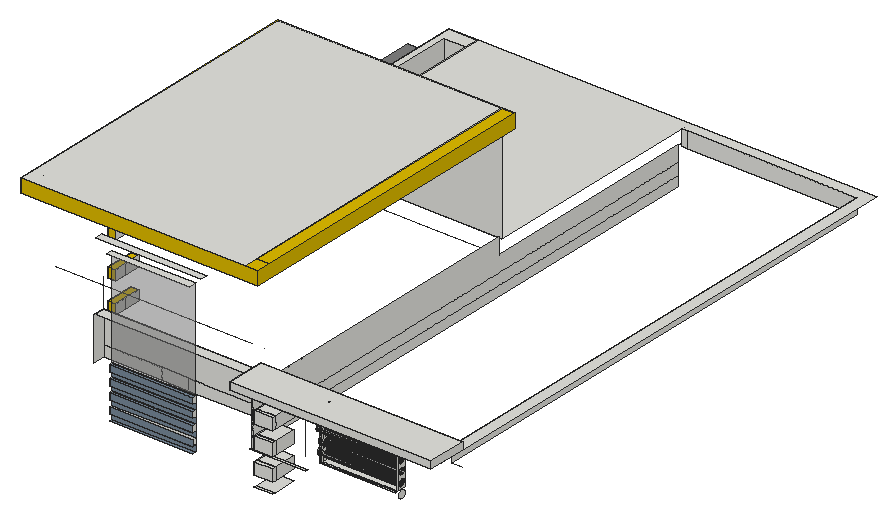
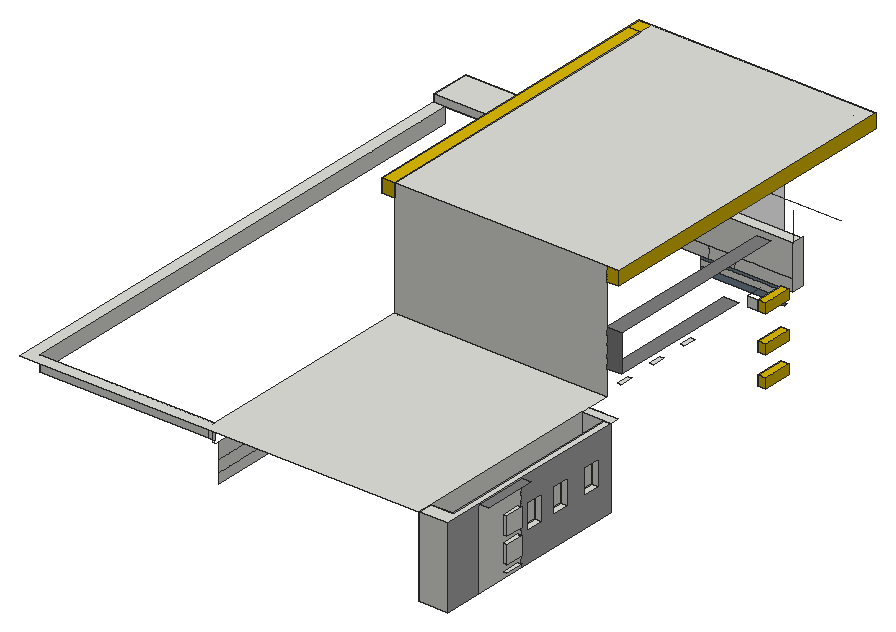
# SketchUp Ruby script. Lengths in inches.
U = 1.inch
M = Sketchup.active_model
def pt(a) = Geom::Point3d.new(a.map { |v| v * U })
def face(e, loops, mat)
  f = e.add_face(loops[0].map { |a| pt(a) })
  loops[1..].each { |l| e.add_face(l.map { |a| pt(a) }).erase! }
  f.material = f.back_material = mat if mat
  f
end
# faces: each face lists its corners as indices into pts; further lists are holes
def faces(e, pts, list, mat = nil) = list.each { |f| face(e, (f[0].is_a?(Array) ? f : [f]).map { |l| l.map { |i| pts[i] } }, mat) }
# xy, xz, yz: faces in a plane at the given z, y or x. An outline is a flat list of corners, or four numbers for a rectangle; further outlines are holes
def ring(l) = l.size == 4 ? [[l[0], l[1]], [l[2], l[1]], [l[2], l[3]], [l[0], l[3]]] : l.each_slice(2).to_a
def flat(e, list, mat, &to3) = list.each { |f| face(e, (f[0].is_a?(Array) ? f : [f]).map { |l| ring(l).map { |u, v| to3.(u, v) } }, mat) }
def xy(e, z, list, mat = nil) = flat(e, list, mat) { |x, y| [x, y, z] }
def xz(e, y, list, mat = nil) = flat(e, list, mat) { |x, z| [x, y, z] }
def yz(e, x, list, mat = nil) = flat(e, list, mat) { |y, z| [x, y, z] }
def lines(e, pts, list) = list.each { |a, b| e.add_line(pt(pts[a]), pt(pts[b])) }
# prism: a flat outline (further loops are holes) pulled along v
def prism(e, loops, v, mat = nil)
  f = face(e, loops, mat); d = Geom::Vector3d.new(v.map { |x| x * U })
  f.pushpull(f.normal.samedirection?(d) ? d.length : -d.length)
end
def box(e, o, s, mat = nil) = prism(e, [[o, [o[0] + s[0], o[1], o[2]], [o[0] + s[0], o[1] + s[1], o[2]], [o[0], o[1] + s[1], o[2]]]], [0, 0, s[2]], mat)
def at(x, y, z, deg = 0) = Geom::Transformation.translation(pt([x, y, z])) * Geom::Transformation.rotation(ORIGIN, Z_AXIS, deg.degrees)
def axes(o, x, y, z) = Geom::Transformation.new([*x, 0, *y, 0, *z, 0, *pt(o).to_a, 1])
def part(name) = M.definitions.add(name)
# library, detail: a bought-in or finely detailed component or shape, given as its bounding box
def library(name, o, s) = part(name).tap { |d| box(d.entities, o, s) }
def detail(e, o, s) = box(e.add_group.entities, o, s)
def put(e, d, t, mat = nil) = e.add_instance(d, t).tap { |i| i.material = mat if mat }
def group(e, t, mat = nil) = e.add_group.tap { |g| g.transformation = t; g.material = mat if mat }.entities
root = M.entities
M.materials.add("[0046_Gold]").color = [221, 186, 0]
M.materials.add("[0110_LightSlateGray]").color = [119, 136, 153]
M.materials.add("[0132_LightGray]").color = [169, 169, 169]
M.materials.add("[0133_Gray]").color = [128, 128, 128]
M.materials.add("[Translucent Glass Gray]").color = [128, 128, 128]
M.materials["[Translucent Glass Gray]"].alpha = 0.5
xy(root,272.6,[[82,329.95,87.58,329.95,87.58,486.08,106,486.08,106,494.21,82,494.21],[87.58,329.95,106,486.08],[82,494.21,106,498.31]])
xy(root,273.2,[[288.75,38.62,303.875,41.62],[288.75,41.62,303.875,61.06]])
xy(root,274.59,[[162.79,46.06,231.72,49.06]],"[0110_LightSlateGray]")
xy(root,280.11,[[162.79,46.06,231.72,49.06]],"[0110_LightSlateGray]")
xy(root,282.14,[[288.75,38.62,303.875,41.62],[288.75,41.62,303.875,61.06]])
xy(root,285.27,[[70.87,436.12,73.87,451.12]])
xy(root,289.0625,[[88,138.31,94,162.08]],"[0046_Gold]")
xy(root,290.55,[[162.79,46.06,231.72,49.06]],"[0110_LightSlateGray]")
xy(root,291.33,[[70.87,436.12,73.87,451.12]])
xy(root,292.2,[[288.75,38.62,303.875,41.62],[288.75,41.62,303.875,61.06]])
xy(root,294.8125,[[279.43,45.87,325.52,47.62],[325.52,60.18,326.02,61.06],[326.02,60.18,388.7,61.06],[325.52,61.06,326.02,70.06],[326.02,61.06,388.7,62.68],
  [326.02,62.68,388.7,70.06]])
xy(root,295.46,[[162.79,46.06,231.72,49.06]],"[0110_LightSlateGray]")
xy(root,297.34,[[88,138.31,94,162.08]],"[0046_Gold]")
xy(root,297.7,[[82,342.29,87.58,357.98],[82,374.54,87.58,390.23],[82,401.35,87.58,417.04]])
xy(root,300.98,[[162.79,46.06,231.72,49.06]],"[0110_LightSlateGray]")
xy(root,301.14,[[288.75,38.62,303.875,41.62],[288.75,41.62,303.875,61.06]])
xy(root,305.9,[[162.79,46.06,231.72,49.06]],"[0110_LightSlateGray]")
xy(root,306.33,[[70.87,436.12,73.87,451.12]])
xy(root,311.2,[[288.75,38.62,303.875,41.62],[288.75,41.62,303.875,61.06]])
xy(root,311.42,[[162.79,46.06,231.72,49.06]],"[0110_LightSlateGray]")
xy(root,312.39,[[70.87,436.12,73.87,451.12]])
xy(root,314.34,[[88,138.31,94,162.08]],"[0046_Gold]")
xy(root,316.34,[[162.79,46.06,231.72,49.06]],"[0110_LightSlateGray]")
xy(root,318.45,[[82,342.29,87.58,357.98],[82,374.54,87.58,390.23],[82,401.35,87.58,417.04]])
xy(root,320.14,[[288.75,38.62,303.875,41.62],[288.75,41.62,303.875,61.06]])
xy(root,322.62,[[88,138.31,94,162.08]],"[0046_Gold]")
xy(root,327.39,[[70.87,436.12,73.87,451.12]])
xy(root,330.2,[[288.75,38.62,303.875,41.62],[288.75,41.62,303.875,61.06]])
xy(root,339,[[269.16,37.37,326.02,41.62],[326.02,37.37,326.02,70.06,388.7,70.06,388.7,47.37,411.96,47.37,411.96,55.06,416.22,55.06,416.22,47.37,436.31,47.37,436.31,37.37],[269.16,41.62,279.47,47.62],[279.47,41.62,288.87,47.62],[288.87,41.62,326.02,47.62],
  [388.7,47.37,411.96,61.68],[416.22,47.37,427.31,48.18],[427.31,47.37,436.31,48.18],[269.16,47.62,279.43,49.06],[279.43,47.62,279.47,49.06],
  [279.47,47.62,288.87,47.62,288.87,56.62,287.5,56.62,287.5,49.06,282.09,49.06,282.09,56.62,279.47,56.62],[288.87,47.62,325.52,56.62],[325.52,47.62,326.02,56.62],[416.22,48.18,427.31,61.06],[427.31,48.18,436.31,61.06],
  [269.16,49.06,279.43,56.62],[279.43,49.06,279.47,56.62],[282.09,49.06,287.5,56.62],[282.09,49.06,287.5,56.62],[411.96,55.06,416.22,61.06],
  [269.16,56.62,279.43,61.06],[279.43,56.62,279.47,60.18],[279.47,56.62,282.09,60.18],[282.09,56.62,287.5,60.18],[287.5,56.62,288.87,60.18],
  [288.87,56.62,325.52,60.18],[325.52,56.62,326.02,60.18],[279.43,60.18,279.47,61.06],[279.47,60.18,282.09,60.81],[282.09,60.18,287.5,60.81],
  [287.5,60.18,288.87,60.81],[288.87,60.18,325.52,60.81],[325.52,60.18,326.02,60.81],[279.47,60.81,282.09,61.06],[282.09,60.81,287.5,61.06],
  [287.5,60.81,288.87,61.06],[288.87,60.81,313.39,61.06],[313.39,60.81,325.52,61.06],[325.52,60.81,326.02,61.06],[138.64,61.06,269.16,70.06],
  [269.16,61.06,279.43,70.06],[279.43,61.06,279.47,70.06],[279.47,61.06,282.09,61.18],[282.09,61.06,287.5,61.18],[287.5,61.06,288.87,61.18],
  [288.87,61.06,313.39,61.18],[313.39,61.06,325.52,61.18],[325.52,61.06,326.02,61.18],[411.96,61.06,416.22,62.68],[416.22,61.06,427.31,62.68],
  [427.31,61.06,436.31,70.06],[279.47,61.18,282.09,61.31],[282.09,61.18,287.5,61.31],[287.5,61.18,288.87,61.31],[288.87,61.18,313.39,61.31],
  [313.39,61.18,325.52,61.31],[325.52,61.18,326.02,61.31],[279.47,61.31,282.09,62.68],[282.09,61.31,287.5,62.68],[287.5,61.31,288.87,62.68],
  [288.87,61.31,313.39,62.68],[313.39,61.31,325.52,62.68],[325.52,61.31,326.02,62.68],[388.7,61.68,411.96,62.68],[279.47,62.68,282.09,70.06],
  [282.09,62.68,287.5,70.06],[287.5,62.68,313.39,70.06],[313.39,62.68,325.52,70.06],[325.52,62.68,326.02,70.06],[388.7,62.68,411.96,70.06],
  [411.96,62.68,416.22,70.06],[416.22,62.68,427.31,70.06],[427.31,70.06,436.31,70.06,436.31,498.31,106,498.31,106,303.56,282.09,303.56,282.09,489.31,427.31,489.31],[279.43,70.06,279.47,303.56],[82,322.08,106,329.95],
  [82,329.95,87.58,329.95,87.58,486.08,106,486.08,106,498.31,82,498.31]])
xy(root,339,[[73.87,422.6,82,466.21]],"[0133_Gray]")
xy(root,341.65,[[106,212.89,109,223.64],[106,244.77,109,255.52],[106,278.27,109,289.02]])
xy(root,344.71,[[88,138.31,94,162.08]],"[0046_Gold]")
xy(root,345,[[269.16,37.37,436.31,70.06]])
xy(root,352.99,[[88,138.31,94,162.08]],"[0046_Gold]")
xy(root,359.72,[[94,182.43,106,303.56]],"[0133_Gray]")
xy(root,390.53,[[94,148.68,106,303.56]],"[0133_Gray]")
xy(root,399.9,[[162.79,43.06,231.72,49.06]])
xy(root,408.9,[[153.79,43.06,240.72,49.06]])
xy(root,424.32,[[103,82.06,106,90.88],[103,99.88,106,108.69],[103,116.44,106,125.25],[106,116.44,109,125.25]])
xy(root,424.32,[[96.18,37.06,96.18,303.56,106,303.56,106,125.25,103,125.25,103,116.44,106,116.44,106,108.69,103,108.69,103,99.88,106,99.88,106,90.88,103,90.88,103,82.06,106,82.06,106,49.06,282.09,49.06,282.09,303.56,292.72,303.56,292.72,37.06]],"[0046_Gold]")
xy(root,435.8125,[[96.18,37.06,282.09,303.56]])
xy(root,435.8125,[[282.09,37.06,292.72,49.06],[282.09,49.06,292.72,303.56]],"[0046_Gold]")
xz(root,37.06,[[96.18,424.32,292.72,435.8125]],"[0046_Gold]")
xz(root,37.37,[[269.16,339,436.31,345]])
xz(root,38.62,[[288.75,282.14,303.875,292.2],[288.75,301.14,303.875,311.2],[288.75,320.14,303.875,330.2]])
xz(root,41.62,[[288.75,282.14,303.875,292.2],[288.75,301.14,303.875,311.2],[288.75,320.14,303.875,330.2]])
xz(root,46.06,[[162.79,280.11,231.72,285.03],[162.79,290.55,231.72,295.46],[162.79,300.98,231.72,305.9],[162.79,311.42,231.72,316.34]],"[0110_LightSlateGray]")
xz(root,49.06,[[162.79,280.11,231.72,285.03],[162.79,290.55,231.72,295.46],[162.79,300.98,231.72,305.9],[162.79,311.42,231.72,316.34]])
xz(root,49.06,[[162.79,274.59,231.72,280.11],[162.79,285.03,231.72,290.55],[162.79,295.46,231.72,300.98],[162.79,305.9,231.72,311.42]],"[0110_LightSlateGray]")
xz(root,49.06,[[162.79,316.34,231.72,399.9]],"[Translucent Glass Gray]")
xz(root,61.06,[[269.16,312.4375,279.43,339]])
xz(root,70.06,[[325.52,294.8125,326.02,339],[138.64,303,186.6,312.4375],[186.6,303,208.53,312.4375],[208.53,303,269.16,312.4375],[138.64,312.4375,269.16,339],
  [269.16,339,436.31,345]])
xz(root,138.31,[[88,289.0625,94,297.34],[88,314.34,94,322.62],[88,344.71,94,352.99]],"[0046_Gold]")
xz(root,162.08,[[94,344.71,103,352.99]])
xz(root,162.08,[[88,289.0625,94,297.34],[88,314.34,94,322.62],[88,344.71,94,352.99]],"[0046_Gold]")
xz(root,303.56,[[106,339,282.09,435.8125]])
xz(root,303.56,[[96.18,424.32,106,435.8125],[282.09,424.32,292.72,435.8125]],"[0046_Gold]")
xz(root,303.56,[[94,359.72,106,390.53]],"[0133_Gray]")
xz(root,329.95,[[82,272.6,87.58,339],[87.58,272.6,106,339]])
xz(root,342.29,[[82,297.7,87.58,318.45]])
xz(root,357.98,[[82,297.7,87.58,318.45]])
xz(root,374.54,[[82,297.7,87.58,318.45]])
xz(root,390.23,[[82,297.7,87.58,318.45]])
xz(root,401.35,[[82,297.7,87.58,318.45]])
xz(root,417.04,[[82,297.7,87.58,318.45]])
xz(root,436.12,[[70.87,291.33,73.87,306.33],[70.87,312.39,73.87,327.39]])
xz(root,451.12,[[70.87,291.33,73.87,306.33],[70.87,312.39,73.87,327.39]])
xz(root,486.08,[[87.58,272.6,106,339]])
xz(root,489.31,[[282.09,325.9375,287.5,339],[287.5,325.9375,427.31,339]])
xz(root,498.31,[[82,272.6,106,339]])
yz(root,70.87,[[436.12,291.33,451.12,306.33],[436.12,312.39,451.12,327.39]])
yz(root,82,[[422.6,272.6,466.21,339]])
yz(root,82,[[[329.95,272.6,422.6,339],[342.29,297.7,357.98,318.45],[374.54,297.7,390.23,318.45],[401.35,297.7,417.04,318.45]],[466.21,272.6,498.31,339]],"[0132_LightGray]")
yz(root,87.58,[[[329.95,272.6,486.08,339],[342.29,297.7,357.98,318.45],[374.54,297.7,390.23,318.45],[401.35,297.7,417.04,318.45]]])
yz(root,88,[[138.31,289.0625,162.08,297.34],[138.31,314.34,162.08,322.62],[138.31,344.71,162.08,352.99]],"[0046_Gold]")
yz(root,94,[[138.31,289.0625,148.68,297.34],[148.68,289.0625,162.08,297.34],[138.31,314.34,148.68,322.62],[148.68,314.34,162.08,322.62],[138.31,344.71,148.68,352.99],
  [148.68,344.71,162.08,352.99]])
yz(root,96.18,[[37.06,424.32,303.56,435.8125]],"[0046_Gold]")
yz(root,106,[[329.95,272.6,486.08,339],[486.08,272.6,498.31,339]])
yz(root,138.64,[[60.43,303,70.06,339]])
yz(root,162.79,[[46.06,280.11,49.06,285.03],[46.06,290.55,49.06,295.46],[46.06,300.98,49.06,305.9],[46.06,311.42,49.06,316.34]])
yz(root,231.72,[[46.06,290.55,49.06,295.46],[46.06,300.98,49.06,305.9],[46.06,311.42,49.06,316.34]])
yz(root,269.16,[[37.37,339,49.06,345],[49.06,339,70.06,345]])
yz(root,279.43,[[47.62,294.8125,49.06,303],[49.06,294.8125,60.18,303],[60.18,294.8125,61.06,303],[61.06,294.8125,489.31,303],[47.62,303,49.06,312.4375],
  [49.06,303,60.18,312.4375],[60.18,303,61.06,312.4375],[61.06,303,489.31,312.4375],[47.62,312.4375,49.06,339],[49.06,312.4375,60.18,339],
  [60.18,312.4375,61.06,339],[61.06,312.4375,489.31,312.4375,489.31,325.9375,303.56,325.9375,303.56,339,61.06,339]])
yz(root,282.09,[[49.06,424.32,303.56,435.8125]])
yz(root,288.75,[[38.62,282.14,41.62,292.2],[41.62,282.14,61.06,292.2],[38.62,301.14,41.62,311.2],[41.62,301.14,61.06,311.2],[38.62,320.14,41.62,330.2],
  [41.62,320.14,61.06,330.2]])
yz(root,292.72,[[37.06,424.32,303.56,435.8125]],"[0046_Gold]")
yz(root,303.875,[[38.62,282.14,41.62,292.2],[41.62,282.14,61.06,292.2],[38.62,301.14,41.62,311.2],[41.62,301.14,61.06,311.2],[38.62,320.14,41.62,330.2],
  [41.62,320.14,61.06,330.2]])
yz(root,320.2,[[66.52,313.71,65.73,313.8125,64.99,314.12,64.36,314.61,63.87,315.24,63.5625,315.98,63.46,316.77,63.5625,317.56,63.87,318.3,64.36,318.9375,64.99,319.42,65.73,319.73,66.52,319.83,67.3125,319.73,68.05,319.42,68.6875,318.9375,69.17,318.3,69.48,317.56,69.58,316.77,69.48,315.98,69.17,315.24,68.6875,314.61,68.05,314.12,67.3125,313.8125]])
yz(root,321.45,[[66.52,296.46,65.73,296.5625,64.99,296.87,64.36,297.36,63.87,297.99,63.5625,298.73,63.46,299.52,63.5625,300.31,63.87,301.05,64.36,301.6875,64.99,302.17,65.73,302.48,66.52,302.58,67.3125,302.48,68.05,302.17,68.6875,301.6875,69.17,301.05,69.48,300.31,69.58,299.52,69.48,298.73,69.17,297.99,68.6875,297.36,68.05,296.87,67.3125,296.5625]])
yz(root,321.52,[[66.52,322.33,65.73,322.4375,64.99,322.74,64.36,323.23,63.87,323.87,63.5625,324.6,63.46,325.4,63.5625,326.19,63.87,326.93,64.36,327.5625,64.99,328.05,65.73,328.36,66.52,328.46,67.3125,328.36,68.05,328.05,68.6875,327.5625,69.17,326.93,69.48,326.19,69.58,325.4,69.48,324.6,69.17,323.87,68.6875,323.23,68.05,322.74,67.3125,322.4375]])
yz(root,322.14,[[66.52,305.08,65.73,305.1875,64.99,305.49,64.36,305.98,63.87,306.62,63.5625,307.35,63.46,308.15,63.5625,308.94,63.87,309.68,64.36,310.3125,64.99,310.8,65.73,311.11,66.52,311.21,67.3125,311.11,68.05,310.8,68.6875,310.3125,69.17,309.68,69.48,308.94,69.58,308.15,69.48,307.35,69.17,306.62,68.6875,305.98,68.05,305.49,67.3125,305.1875]])
yz(root,326.02,[[60.18,294.8125,60.81,339],[60.81,294.8125,61.06,339],[61.06,294.8125,61.18,339],[61.18,294.8125,61.31,339],[61.31,294.8125,62.68,339],
  [62.68,294.8125,70.06,339]])
yz(root,388.7,[[66.52,287.83,65.73,287.9375,64.99,288.24,64.36,288.73,63.87,289.37,63.5625,290.1,63.46,290.9,63.5625,291.69,63.87,292.43,64.36,293.0625,64.99,293.55,65.73,293.86,66.52,293.96,67.3125,293.86,68.05,293.55,68.6875,293.0625,69.17,292.43,69.48,291.69,69.58,290.9,69.48,290.1,69.17,289.37,68.6875,288.73,68.05,288.24,67.3125,287.9375],[61.68,294.8125,62.68,339],[[62.68,294.8125,70.06,339],[66.52,322.33,67.3125,322.4375,68.05,322.74,68.6875,323.23,69.17,323.87,69.48,324.6,69.58,325.4,69.48,326.19,69.17,326.93,68.6875,327.5625,68.05,328.05,67.3125,328.36,66.52,328.46,65.73,328.36,64.99,328.05,64.36,327.5625,63.87,326.93,63.5625,326.19,63.46,325.4,63.5625,324.6,63.87,323.87,64.36,323.23,64.99,322.74,65.73,322.4375],[66.52,313.71,67.3125,313.8125,68.05,314.12,68.6875,314.61,69.17,315.24,69.48,315.98,69.58,316.77,69.48,317.56,69.17,318.3,68.6875,318.9375,68.05,319.42,67.3125,319.73,66.52,319.83,65.73,319.73,64.99,319.42,64.36,318.9375,63.87,318.3,63.5625,317.56,63.46,316.77,63.5625,315.98,63.87,315.24,64.36,314.61,64.99,314.12,65.73,313.8125],[66.52,305.08,67.3125,305.1875,68.05,305.49,68.6875,305.98,69.17,306.62,69.48,307.35,69.58,308.15,69.48,308.94,69.17,309.68,68.6875,310.3125,68.05,310.8,67.3125,311.11,66.52,311.21,65.73,311.11,64.99,310.8,64.36,310.3125,63.87,309.68,63.5625,308.94,63.46,308.15,63.5625,307.35,63.87,306.62,64.36,305.98,64.99,305.49,65.73,305.1875],[66.52,296.46,67.3125,296.5625,68.05,296.87,68.6875,297.36,69.17,297.99,69.48,298.73,69.58,299.52,69.48,300.31,69.17,301.05,68.6875,301.6875,68.05,302.17,67.3125,302.48,66.52,302.58,65.73,302.48,64.99,302.17,64.36,301.6875,63.87,301.05,63.5625,300.31,63.46,299.52,63.5625,298.73,63.87,297.99,64.36,297.36,64.99,296.87,65.73,296.5625],[66.52,330.96,67.3125,331.0625,68.05,331.37,68.6875,331.86,69.17,332.49,69.48,333.23,69.58,334.02,69.48,334.81,69.17,335.55,68.6875,336.1875,68.05,336.67,67.3125,336.98,66.52,337.08,65.73,336.98,64.99,336.67,64.36,336.1875,63.87,335.55,63.5625,334.81,63.46,334.02,63.5625,333.23,63.87,332.49,64.36,331.86,64.99,331.37,65.73,331.0625]]])
yz(root,427.31,[[70.06,325.9375,489.31,339]])
yz(root,436.31,[[37.37,339,70.06,345]])
p = [[388.7,66.52,296.46],[388.7,65.73,296.5625],[321.45,65.73,296.5625],[321.45,66.52,296.46],[388.7,67.3125,296.5625],[321.45,67.3125,296.5625],
  [388.7,64.99,296.87],[321.45,64.99,296.87],[388.7,68.05,296.87],[321.45,68.05,296.87],[388.7,64.36,297.36],[321.45,64.36,297.36],
  [388.7,68.6875,297.36],[321.45,68.6875,297.36],[388.7,63.87,297.99],[321.45,63.87,297.99],[388.7,69.17,297.99],[321.45,69.17,297.99],
  [388.7,63.5625,298.73],[321.45,63.5625,298.73],[388.7,69.48,298.73],[321.45,69.48,298.73],[388.7,63.46,299.52],[321.45,63.46,299.52],
  [388.7,69.58,299.52],[321.45,69.58,299.52],[388.7,63.5625,300.31],[321.45,63.5625,300.31],[388.7,69.48,300.31],[321.45,69.48,300.31],
  [388.7,63.87,301.05],[321.45,63.87,301.05],[388.7,69.17,301.05],[321.45,69.17,301.05],[388.7,64.36,301.6875],[321.45,64.36,301.6875],
  [388.7,68.6875,301.6875],[321.45,68.6875,301.6875],[388.7,64.99,302.17],[321.45,64.99,302.17],[388.7,68.05,302.17],[321.45,68.05,302.17],
  [388.7,65.73,302.48],[321.45,65.73,302.48],[388.7,67.3125,302.48],[321.45,67.3125,302.48],[388.7,66.52,302.58],[321.45,66.52,302.58],
  [388.7,66.52,305.08],[388.7,65.73,305.1875],[322.14,65.73,305.1875],[322.14,66.52,305.08],[388.7,67.3125,305.1875],[322.14,67.3125,305.1875],
  [388.7,64.99,305.49],[322.14,64.99,305.49],[388.7,68.05,305.49],[322.14,68.05,305.49],[388.7,64.36,305.98],[322.14,64.36,305.98],
  [388.7,68.6875,305.98],[322.14,68.6875,305.98],[388.7,63.87,306.62],[322.14,63.87,306.62],[388.7,69.17,306.62],[322.14,69.17,306.62],
  [388.7,63.5625,307.35],[322.14,63.5625,307.35],[388.7,69.48,307.35],[322.14,69.48,307.35],[388.7,63.46,308.15],[322.14,63.46,308.15],
  [388.7,69.58,308.15],[322.14,69.58,308.15],[388.7,63.5625,308.94],[322.14,63.5625,308.94],[388.7,69.48,308.94],[322.14,69.48,308.94],
  [388.7,63.87,309.68],[322.14,63.87,309.68],[388.7,69.17,309.68],[322.14,69.17,309.68],[388.7,64.36,310.3125],[322.14,64.36,310.3125],
  [388.7,68.6875,310.3125],[322.14,68.6875,310.3125],[388.7,64.99,310.8],[322.14,64.99,310.8],[388.7,68.05,310.8],[322.14,68.05,310.8],
  [388.7,65.73,311.11],[322.14,65.73,311.11],[388.7,67.3125,311.11],[322.14,67.3125,311.11],[388.7,66.52,311.21],[322.14,66.52,311.21],
  [388.7,66.52,313.71],[388.7,65.73,313.8125],[320.2,65.73,313.8125],[320.2,66.52,313.71],[388.7,67.3125,313.8125],[320.2,67.3125,313.8125],
  [388.7,64.99,314.12],[320.2,64.99,314.12],[388.7,68.05,314.12],[320.2,68.05,314.12],[388.7,64.36,314.61],[320.2,64.36,314.61],
  [388.7,68.6875,314.61],[320.2,68.6875,314.61],[388.7,63.87,315.24],[320.2,63.87,315.24],[388.7,69.17,315.24],[320.2,69.17,315.24],
  [388.7,63.5625,315.98],[320.2,63.5625,315.98],[388.7,69.48,315.98],[320.2,69.48,315.98],[388.7,63.46,316.77],[320.2,63.46,316.77],
  [388.7,69.58,316.77],[320.2,69.58,316.77],[388.7,63.5625,317.56],[320.2,63.5625,317.56],[388.7,69.48,317.56],[320.2,69.48,317.56],
  [388.7,63.87,318.3],[320.2,63.87,318.3],[388.7,69.17,318.3],[320.2,69.17,318.3],[388.7,64.36,318.9375],[320.2,64.36,318.9375],
  [388.7,68.6875,318.9375],[320.2,68.6875,318.9375],[388.7,64.99,319.42],[320.2,64.99,319.42],[388.7,68.05,319.42],[320.2,68.05,319.42],
  [388.7,65.73,319.73],[320.2,65.73,319.73],[388.7,67.3125,319.73],[320.2,67.3125,319.73],[388.7,66.52,319.83],[320.2,66.52,319.83],
  [388.7,66.52,322.33],[388.7,65.73,322.4375],[321.52,65.73,322.4375],[321.52,66.52,322.33],[388.7,67.3125,322.4375],[321.52,67.3125,322.4375],
  [388.7,64.99,322.74],[321.52,64.99,322.74],[388.7,68.05,322.74],[321.52,68.05,322.74],[388.7,64.36,323.23],[321.52,64.36,323.23],
  [388.7,68.6875,323.23],[321.52,68.6875,323.23],[388.7,63.87,323.87],[321.52,63.87,323.87],[388.7,69.17,323.87],[321.52,69.17,323.87],
  [388.7,63.5625,324.6],[321.52,63.5625,324.6],[388.7,69.48,324.6],[321.52,69.48,324.6],[388.7,63.46,325.4],[321.52,63.46,325.4],
  [388.7,69.58,325.4],[321.52,69.58,325.4],[388.7,63.5625,326.19],[321.52,63.5625,326.19],[388.7,69.48,326.19],[321.52,69.48,326.19],
  [388.7,63.87,326.93],[321.52,63.87,326.93],[388.7,69.17,326.93],[321.52,69.17,326.93],[388.7,64.36,327.5625],[321.52,64.36,327.5625],
  [388.7,68.6875,327.5625],[321.52,68.6875,327.5625],[388.7,64.99,328.05],[321.52,64.99,328.05],[388.7,68.05,328.05],[321.52,68.05,328.05],
  [388.7,65.73,328.36],[321.52,65.73,328.36],[388.7,67.3125,328.36],[321.52,67.3125,328.36],[388.7,66.52,328.46],[321.52,66.52,328.46],
  [388.7,66.52,330.96],[388.7,65.73,331.0625],[326.02,65.73,331.0625],[326.02,66.52,330.96],[388.7,67.3125,331.0625],[326.02,67.3125,331.0625],
  [388.7,64.99,331.37],[326.02,64.99,331.37],[388.7,68.05,331.37],[326.02,68.05,331.37],[388.7,64.36,331.86],[326.02,64.36,331.86],
  [388.7,68.6875,331.86],[326.02,68.6875,331.86],[388.7,63.87,332.49],[326.02,63.87,332.49],[388.7,69.17,332.49],[326.02,69.17,332.49],
  [388.7,63.5625,333.23],[326.02,63.5625,333.23],[388.7,69.48,333.23],[326.02,69.48,333.23],[388.7,63.46,334.02],[326.02,63.46,334.02],
  [388.7,69.58,334.02],[326.02,69.58,334.02],[388.7,63.5625,334.81],[326.02,63.5625,334.81],[388.7,69.48,334.81],[326.02,69.48,334.81],
  [388.7,63.87,335.55],[326.02,63.87,335.55],[388.7,69.17,335.55],[326.02,69.17,335.55],[388.7,64.36,336.1875],[326.02,64.36,336.1875],
  [388.7,68.6875,336.1875],[326.02,68.6875,336.1875],[388.7,64.99,336.67],[326.02,64.99,336.67],[388.7,68.05,336.67],[326.02,68.05,336.67],
  [388.7,65.73,336.98],[326.02,65.73,336.98],[388.7,67.3125,336.98],[326.02,67.3125,336.98],[388.7,66.52,337.08],[326.02,66.52,337.08],
  [279.43,60.93,363],[279.43,61.06,363],[269.16,61.06,363],[106,61.06,363],[138.64,70.06,339],[138.64,70.06,363],
  [313.39,61.06,294.8125],[313.39,61.06,339],[282.09,489.31,325.9375],[282.09,491.93,325.9375],[279.43,491.93,325.9375],[279.43,489.31,325.9375],
  [279.43,303.56,325.9375],[106,303.56,325.9375],[427.31,70.06,325.9375],[436.31,70.06,325.9375],[282.09,491.93,339],[106,49.06,435.8125],
  [106,49.06,424.32],[103,162.08,352.99],[103,148.68,352.99],[103,148.68,344.71],[103,162.08,344.71]]
faces(root,p,[[0,1,2,3],[4,0,3,5],[1,6,7,2],[8,4,5,9],[6,10,11,7],[12,8,9,13],[10,14,15,11],[16,12,13,17],
  [14,18,19,15],[20,16,17,21],[18,22,23,19],[24,20,21,25],[22,26,27,23],[28,24,25,29],[26,30,31,27],[32,28,29,33],
  [30,34,35,31],[36,32,33,37],[34,38,39,35],[40,36,37,41],[38,42,43,39],[44,40,41,45],[42,46,47,43],[46,44,45,47],
  [48,49,50,51],[52,48,51,53],[49,54,55,50],[56,52,53,57],[54,58,59,55],[60,56,57,61],[58,62,63,59],[64,60,61,65],
  [62,66,67,63],[68,64,65,69],[66,70,71,67],[72,68,69,73],[70,74,75,71],[76,72,73,77],[74,78,79,75],[80,76,77,81],
  [78,82,83,79],[84,80,81,85],[82,86,87,83],[88,84,85,89],[86,90,91,87],[92,88,89,93],[90,94,95,91],[94,92,93,95],
  [96,97,98,99],[100,96,99,101],[97,102,103,98],[104,100,101,105],[102,106,107,103],[108,104,105,109],[106,110,111,107],[112,108,109,113],
  [110,114,115,111],[116,112,113,117],[114,118,119,115],[120,116,117,121],[118,122,123,119],[124,120,121,125],[122,126,127,123],[128,124,125,129],
  [126,130,131,127],[132,128,129,133],[130,134,135,131],[136,132,133,137],[134,138,139,135],[140,136,137,141],[138,142,143,139],[142,140,141,143],
  [144,145,146,147],[148,144,147,149],[145,150,151,146],[152,148,149,153],[150,154,155,151],[156,152,153,157],[154,158,159,155],[160,156,157,161],
  [158,162,163,159],[164,160,161,165],[162,166,167,163],[168,164,165,169],[166,170,171,167],[172,168,169,173],[170,174,175,171],[176,172,173,177],
  [174,178,179,175],[180,176,177,181],[178,182,183,179],[184,180,181,185],[182,186,187,183],[188,184,185,189],[186,190,191,187],[190,188,189,191],
  [192,193,194,195],[196,192,195,197],[193,198,199,194],[200,196,197,201],[198,202,203,199],[204,200,201,205],[202,206,207,203],[208,204,205,209],
  [206,210,211,207],[212,208,209,213],[210,214,215,211],[216,212,213,217],[214,218,219,215],[220,216,217,221],[218,222,223,219],[224,220,221,225],
  [222,226,227,223],[228,224,225,229],[226,230,231,227],[232,228,229,233],[230,234,235,231],[236,232,233,237],[234,238,239,235],[238,236,237,239]],"[0132_LightGray]")
lines(root,p,[[240,241],[242,243],[244,245],[246,247],[248,249],[250,249],[250,251],[252,253],[254,255],[256,249],[257,258],[259,260],
  [261,262]])
